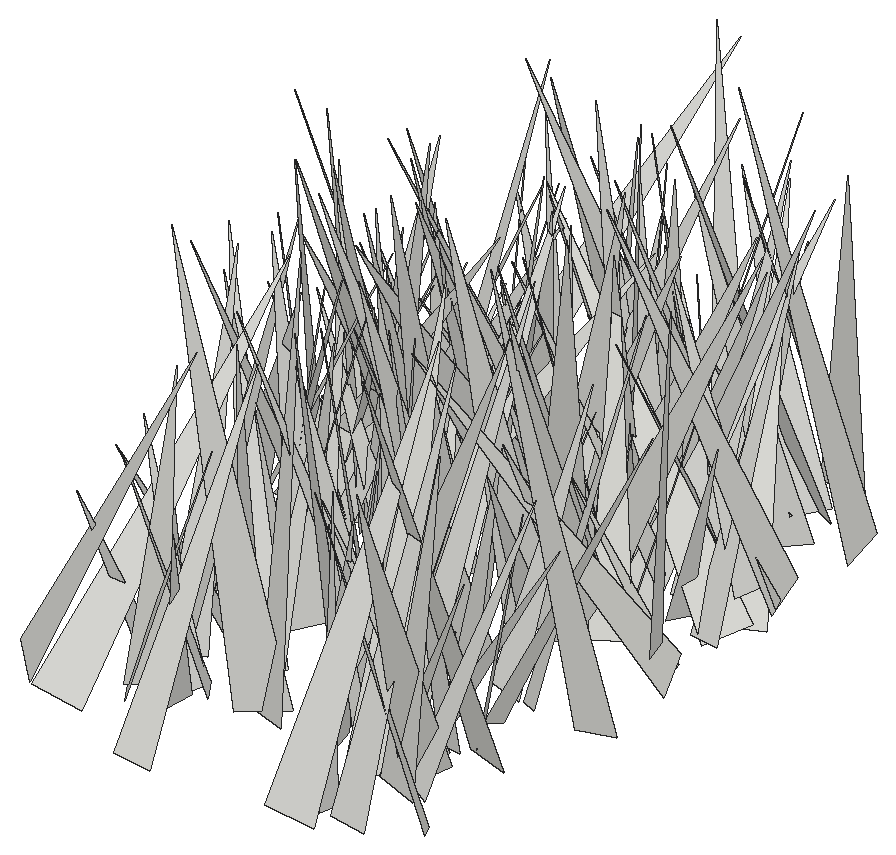
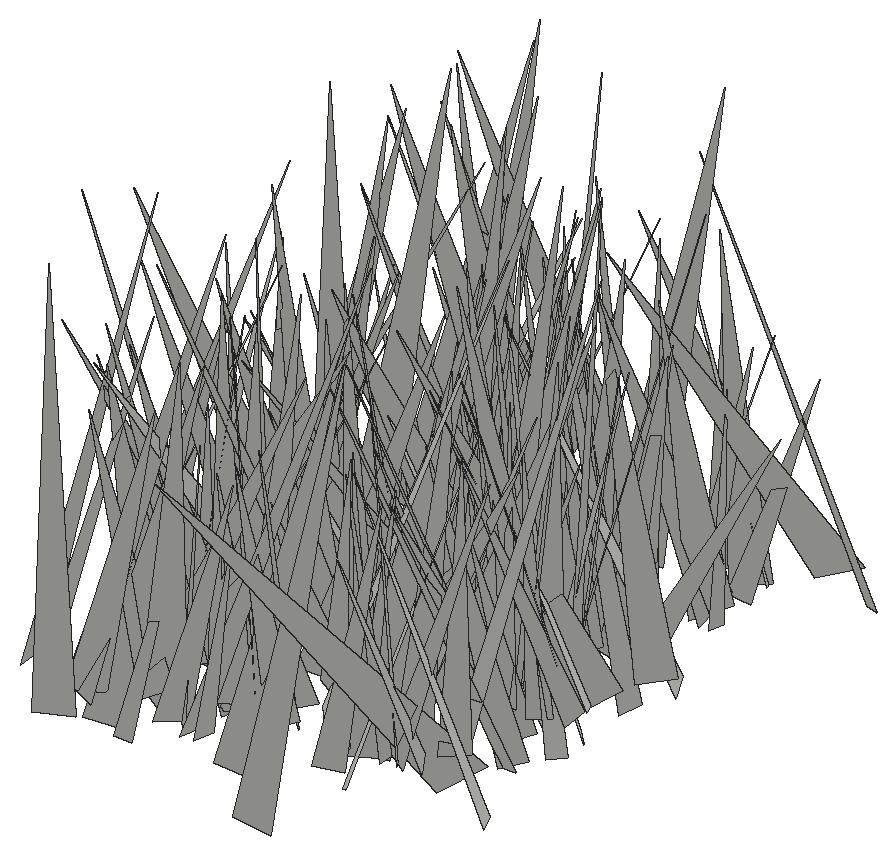
# SketchUp Ruby script. Lengths in inches.
U = 1.inch
M = Sketchup.active_model
def pt(a) = Geom::Point3d.new(a.map { |v| v * U })
def face(e, loops, mat)
  f = e.add_face(loops[0].map { |a| pt(a) })
  loops[1..].each { |l| e.add_face(l.map { |a| pt(a) }).erase! }
  f.material = f.back_material = mat if mat
  f
end
# faces: each face lists its corners as indices into pts; further lists are holes
def faces(e, pts, list, mat = nil) = list.each { |f| face(e, (f[0].is_a?(Array) ? f : [f]).map { |l| l.map { |i| pts[i] } }, mat) }
# xy, xz, yz: faces in a plane at the given z, y or x. An outline is a flat list of corners, or four numbers for a rectangle; further outlines are holes
def ring(l) = l.size == 4 ? [[l[0], l[1]], [l[2], l[1]], [l[2], l[3]], [l[0], l[3]]] : l.each_slice(2).to_a
def flat(e, list, mat, &to3) = list.each { |f| face(e, (f[0].is_a?(Array) ? f : [f]).map { |l| ring(l).map { |u, v| to3.(u, v) } }, mat) }
def xy(e, z, list, mat = nil) = flat(e, list, mat) { |x, y| [x, y, z] }
def xz(e, y, list, mat = nil) = flat(e, list, mat) { |x, z| [x, y, z] }
def yz(e, x, list, mat = nil) = flat(e, list, mat) { |y, z| [x, y, z] }
def lines(e, pts, list) = list.each { |a, b| e.add_line(pt(pts[a]), pt(pts[b])) }
# prism: a flat outline (further loops are holes) pulled along v
def prism(e, loops, v, mat = nil)
  f = face(e, loops, mat); d = Geom::Vector3d.new(v.map { |x| x * U })
  f.pushpull(f.normal.samedirection?(d) ? d.length : -d.length)
end
def box(e, o, s, mat = nil) = prism(e, [[o, [o[0] + s[0], o[1], o[2]], [o[0] + s[0], o[1] + s[1], o[2]], [o[0], o[1] + s[1], o[2]]]], [0, 0, s[2]], mat)
def at(x, y, z, deg = 0) = Geom::Transformation.translation(pt([x, y, z])) * Geom::Transformation.rotation(ORIGIN, Z_AXIS, deg.degrees)
def axes(o, x, y, z) = Geom::Transformation.new([*x, 0, *y, 0, *z, 0, *pt(o).to_a, 1])
def part(name) = M.definitions.add(name)
# library, detail: a bought-in or finely detailed component or shape, given as its bounding box
def library(name, o, s) = part(name).tap { |d| box(d.entities, o, s) }
def detail(e, o, s) = box(e.add_group.entities, o, s)
def put(e, d, t, mat = nil) = e.add_instance(d, t).tap { |i| i.material = mat if mat }
def group(e, t, mat = nil) = e.add_group.tap { |g| g.transformation = t; g.material = mat if mat }.entities
root = M.entities
c1 = part("fur_instance\#9")
p = [[0.8125,0,1.79],[0.67,-0.02,1.48],[0,-0.11,0],[0,0.11,0]]
faces(c1.entities,p,[[0,1,2,3]])
put(root,c1,axes([100.98,190.09,-27.1],[-2.4507,-4.58404,1.24543],[-4.71435,2.17524,-1.27033],[-0.58261,1.68089,5.0404]))
put(root,c1,axes([100.875,177.61,-28.22],[-0.33006,-3.76044,0.39687],[-3.50265,0.15395,-1.45434],[-1.42474,0.49269,3.4835]))
put(root,c1,axes([100.43,182.3,-28.22],[3.89411,3.28531,3.07479],[3.51498,-4.75969,0.63397],[-2.80935,-1.40135,5.05524]))
put(root,c1,axes([100.59,187.69,-28.22],[-4.98525,-6.36904,1.05647],[-6.36247,5.07321,0.56124],[1.09531,0.48105,8.06861]))
put(root,c1,axes([100.27,174.66,-28.22],[0.67909,-3.62862,0.46379],[-3.53581,-0.77205,-0.86319],[-0.93808,0.2832,3.58928]))
put(root,c1,axes([100.42,183.74,-27.1],[-4.38445,3.57185,1.79964],[3.76738,4.58485,0.07863],[1.34299,-1.20052,5.65467]))
put(root,c1,axes([100.8125,183.89,-27.1],[-6.07164,-2.28107,2.04855],[-2.55827,6.27412,-0.5961],[1.68971,1.3026,6.45854]))
put(root,c1,axes([100.88,179.83,-28.22],[-0.52973,-5.32119,2.08202],[-5.65742,0.19488,-0.94137],[-0.8022,2.1395,5.26399]))
put(root,c1,axes([100.17,184.2,-28.22],[-3.60567,-4.25836,0.82426],[-4.10665,3.69659,1.13335],[1.39586,-0.12438,5.46351]))
put(root,c1,axes([97.62,189.9,-28.22],[5.05169,2.87341,0.23488],[2.86098,-4.93803,-1.1233],[0.35552,-1.09113,5.70213]))
put(root,c1,axes([100.38,175.82,-28.22],[-5.11212,3.73872,1.49873],[3.53116,5.32488,-1.23875],[1.93782,0.15985,6.21106]))
put(root,c1,axes([98.25,184.95,-27.1],[4.49912,0.07902,0.02983],[0.07502,-4.46879,0.52292],[-0.03881,0.52233,4.46932]))
put(root,c1,axes([99.66,188.87,-27.1],[-3.20699,2.34244,2.63387],[2.95903,3.72406,0.29089],[1.91533,-1.83124,3.96071]))
put(root,c1,axes([99.71,176.41,-28.22],[3.54062,0.10617,1.20258],[0.38468,-3.63127,-0.812],[-1.14433,-0.89222,3.44788]))
put(root,c1,axes([97.8,181.64,-27.1],[2.89446,-5.47209,0.08006],[-5.31049,-2.7865,1.53693],[1.32243,0.78724,5.99662]))
put(root,c1,axes([99.11,185.56,-27.1],[1.24719,-3.91493,0.4967],[-3.8954,-1.13791,0.81231],[0.63182,0.71228,4.02769]))
put(root,c1,axes([96.81,172.67,-28.22],[5.1253,5.35023,0.94765],[5.22805,-4.50107,-2.86349],[1.48003,-2.62814,6.83331]))
put(root,c1,axes([102.79,176.58,-28.22],[-1.83761,6.5724,0.07775],[6.30696,1.74042,1.94227],[-1.85059,-0.59481,6.54223]))
put(root,c1,axes([100.66,182.59,-28.22],[-6.12859,-4.53414,1.24355],[-3.97845,6.08997,2.59781],[2.50535,-1.42065,7.16724]))
put(root,c1,axes([98.93,171.52,-28.22],[-2.37553,7.32496,0.20013],[6.77476,2.27563,-2.87444],[2.79244,0.71043,7.14393]))
put(root,c1,axes([99.67,183.23,-27.1],[6.5233,2.37968,3.04495],[3.30026,-6.53866,-1.96019],[-2.01069,-3.01183,6.66138]))
put(root,c1,axes([100.63,181.82,-27.1],[-2.63101,2.88231,1.12737],[2.88894,2.81797,-0.46255],[1.11028,-0.50218,3.87505]))
put(root,c1,axes([100.39,175.6,-28.22],[6.48387,0.57283,2.72889],[-0.5216,-6.53637,2.61139],[-2.73914,2.60063,5.96233]))
put(root,c1,axes([100.08,189.85,-27.1],[3.50829,2.33455,0.59392],[2.17247,-3.51961,1.00185],[-1.04078,0.52272,4.09323]))
put(root,c1,axes([100.02,185.17,-28.22],[-2.24113,2.46388,1.48853],[2.36542,2.65133,-0.82724],[1.6405,-0.45695,3.22631]))
put(root,c1,axes([98.65,184.1,-28.22],[4.58071,3.98416,0.78034],[4.05613,-4.44078,-1.1369],[0.17387,-1.36793,5.96354]))
put(root,c1,axes([98.3,179.92,-28.22],[5.74165,3.30721,0.02247],[3.30582,-5.73764,-0.2359],[0.09829,-0.21562,6.62182]))
put(root,c1,axes([98.36,184.14,-27.1],[4.34126,2.62004,0.01209],[2.52851,-4.18338,-1.34808],[0.68659,-1.1602,4.88813]))
put(root,c1,axes([102.34,183.51,-28.22],[-4.67838,0.58429,0.4377],[0.60816,4.68963,0.24018],[0.40387,-0.29353,4.7086]))
put(root,c1,axes([98.58,181.91,-28.22],[6.48852,0.93317,0.66882],[1.0636,-6.33108,-1.48501],[-0.43231,-1.57025,6.38486]))
put(root,c1,axes([101.82,174.375,-28.22],[-4.10178,1.61092,0.95507],[1.70987,4.15942,0.32775],[0.76391,-0.66031,4.39457]))
put(root,c1,axes([100.35,185.52,-27.1],[-1.33091,-4.34516,1.37723],[-4.35803,1.6335,0.94222],[1.33595,0.99989,4.44566]))
put(root,c1,axes([98.46,185.55,-28.22],[6.70588,0.95076,0.50826],[1.07552,-6.12086,-2.74035],[-0.07444,-2.78609,6.19381]))
put(root,c1,axes([101.58,183.73,-28.22],[-4.04138,0.55951,1.25439],[0.25517,4.13619,-1.02282],[1.34961,0.89343,3.94964]))
put(root,c1,axes([101.98,186.08,-27.1],[0.91658,-6.09487,0.23316],[-5.96683,-0.94489,-1.24341],[-1.26442,0.04079,6.03668]))
put(root,c1,axes([100.53,173.76,-28.22],[3.55242,-4.27149,1.91187],[-4.60398,-3.6203,0.46613],[-0.83917,1.77997,5.53606]))
put(root,c1,axes([100.52,181.37,-27.1],[3.76138,-1.24538,0.93866],[-1.27843,-3.86595,-0.00634],[-0.89313,0.28885,3.96218]))
put(root,c1,axes([102.1875,174.68,-28.22],[-3.61255,-2.36918,0.54232],[-2.35627,3.65218,0.25916],[0.59592,0.07847,4.31235]))
put(root,c1,axes([99.2,186.66,-28.22],[1.64693,-4.65446,0.85777],[-4.4282,-1.19483,2.01879],[1.67056,1.42146,4.50564]))
put(root,c1,axes([100.32,183.96,-27.1],[-1.02594,6.32348,2.52203],[6.58274,1.57191,-1.26344],[1.73626,-2.22313,6.28034]))
put(root,c1,axes([101.61,185.42,-27.1],[-1.56855,-7.63886,0.47282],[-7.63369,1.59619,0.46371],[0.55001,0.36889,7.78444]))
put(root,c1,axes([102.1,191.83,-27.1],[1.8151,-3.86013,1.55176],[-3.9232,-2.15155,-0.76319],[-1.38458,1.03602,4.19675]))
put(root,c1,axes([102.1875,179.7,-28.22],[-5.43342,3.18473,2.47254],[3.60205,5.6984,0.57576],[1.81141,-1.77869,6.27161]))
put(root,c1,axes([98.34,183.59,-27.1],[4.70359,-4.43483,0.77561],[-4.1988,-3.91632,3.07011],[1.62462,2.71804,5.6891]))
put(root,c1,axes([103.16,185.85,-27.1],[-3.34237,-3.67886,0.49489],[-3.71061,3.29315,-0.58039],[-0.10119,0.75599,4.93646]))
put(root,c1,axes([100.68,184.72,-28.22],[-0.26739,4.57604,0.32256],[4.40279,0.34673,-1.26925],[1.2883,-0.2352,4.40462]))
put(root,c1,axes([100.87,190.08,-27.1],[4.61711,2.95667,1.94744],[3.35791,-4.67134,-0.86895],[-1.12198,-1.8135,5.41336]))
put(root,c1,axes([103.87,185.64,-27.1],[-0.77186,4.35622,1.72795],[4.2436,-0.09339,2.13104],[-1.98854,-1.8902,3.87699]))
put(root,c1,axes([100.25,180.17,-28.22],[5.36268,3.16176,1.79895],[3.56295,-5.21159,-1.4615],[-0.73371,-2.1986,6.05138]))
put(root,c1,axes([101.04,185.3,-27.1],[-1.24529,-7.71146,0.7872],[-7.61167,1.36728,1.35282],[1.46589,0.54863,7.69333]))
put(root,c1,axes([100.09,182.55,-28.22],[2.55836,5.15566,0.46861],[5.11042,-2.43162,-1.14739],[0.82709,-0.92305,5.63999]))
put(root,c1,axes([99.83,188.29,-28.22],[-4.06981,7.2471,0.38585],[5.9474,3.58401,-4.58433],[4.15906,1.9665,6.9331]))
put(root,c1,axes([100.18,173.33,-28.22],[4.57096,2.53062,0.74602],[2.63797,-4.36083,-1.37058],[0.04077,-1.55993,5.04174]))
put(root,c1,axes([99.12,186.99,-28.22],[3.70489,5.29932,0.63458],[5.07029,-3.25343,-2.43293],[1.66665,-1.88258,5.99082]))
put(root,c1,axes([101.12,183.57,-27.1],[-2.2184,-4.85625,2.50772],[-5.03427,2.86928,1.10295],[2.1279,1.72546,5.22379]))
put(root,c1,axes([101.44,183.625,-28.22],[6.98669,-0.82296,2.45735],[-1.02769,-7.36659,0.45485],[-2.37901,0.76535,7.02027]))
put(root,c1,axes([101.55,177.47,-28.22],[-1.49561,-5.63035,1.67127],[-5.71638,1.79132,0.91926],[1.34798,1.34949,5.75262]))
put(root,c1,axes([102.22,190.92,-28.22],[-3.99829,-3.957,0.07334],[-3.50173,3.58563,2.55553],[1.84422,-1.77059,5.01133]))
put(root,c1,axes([101.11,190.28,-27.1],[4.30698,0.82715,0.77594],[0.97071,-4.26434,-0.84231],[-0.5865,-0.98365,4.30404]))
put(root,c1,axes([101.54,178.26,-28.22],[4.69636,2.95892,0.9191],[2.85112,-4.78039,0.82137],[-1.21287,0.21986,5.48965]))
put(root,c1,axes([102.53,184.15,-27.1],[3.62911,6.60842,0.2466],[6.35712,-3.56375,1.94657],[-1.82181,0.72867,7.28371]))
put(root,c1,axes([101.15,189.01,-27.1],[5.45875,-2.61976,0.1584],[-2.41646,-5.15945,-2.05595],[-1.02417,-1.78972,5.6951]))
put(root,c1,axes([101.06,185.93,-27.1],[1.63148,3.88333,0.8996],[3.80186,-1.22375,-1.61232],[1.19808,-1.40479,3.89132]))
put(root,c1,axes([102.97,194.36,-28.22],[-1.0754,-7.3325,1.08617],[-7.40599,1.10888,0.15329],[0.31086,1.05196,7.40935]))
put(root,c1,axes([101.9375,173.57,-28.22],[3.94789,-1.4658,0.35037],[-1.34081,-3.86465,-1.06014],[-0.68816,-0.87925,4.0756]))
put(root,c1,axes([104.23,174.6875,-28.22],[2.49125,-7.31611,3.2771],[-7.62751,-3.2193,-1.38865],[-2.46697,2.5655,7.60286]))
put(root,c1,axes([103.25,188.63,-27.1],[-1.22069,-3.41408,1.05948],[-3.55821,1.26785,-0.01408],[0.34288,1.00256,3.62571]))
put(root,c1,axes([103.94,184.47,-28.22],[-7.41474,-1.37074,2.09218],[-0.74138,7.45582,2.25736],[2.38883,-1.94072,7.19456]))
put(root,c1,axes([104.77,188.24,-27.1],[1.00631,5.78428,1.17144],[5.41169,-1.37849,2.15781],[-2.35451,-0.6962,5.46025]))
put(root,c1,axes([104.25,189.35,-27.1],[-5.79035,-4.99721,0.36352],[-4.82955,5.71454,1.62848],[1.33407,-1.00217,7.47317]))
put(root,c1,axes([103.11,188.89,-28.22],[2.31085,-7.14722,0.11909],[-7.10013,-2.30949,-0.83147],[-0.82765,-0.14321,7.46535]))
put(root,c1,axes([103.4,184.15,-27.1],[-5.97447,-2.65496,2.2585],[-2.10106,6.3191,1.8704],[2.78122,-0.92951,6.26456]))
put(root,c1,axes([104.46,185.94,-27.1],[-2.38494,-6.16406,1.52656],[-6.35023,2.30898,-0.59758],[-0.0234,1.63919,6.58229]))
put(root,c1,axes([103.66,184.99,-28.22],[1.41164,-4.04262,0.99191],[-4.10193,-1.52908,-0.39425],[-0.70768,0.79907,4.26381]))
put(root,c1,axes([103.11,169.86,-28.22],[0.40052,6.46259,0.29319],[6.45769,-0.38185,-0.40475],[0.38629,-0.31712,6.46233]))
put(root,c1,axes([104.18,181.32,-28.22],[-6.58404,0.20466,2.39247],[0.20033,7.00521,-0.04793],[2.39284,-0.02336,6.58705]))
put(root,c1,axes([103.93,182.38,-27.1],[-0.42673,3.51272,1.26133],[3.73148,0.37463,0.21911],[-0.0791,-1.27778,3.53176]))
put(root,c1,axes([104.52,182.29,-28.22],[-3.06168,2.49465,0.02952],[2.42804,2.99025,-0.87237],[0.57338,0.65813,3.85176]))
put(root,c1,axes([103.3125,188.57,-27.1],[-0.92871,-3.83483,1.6083],[-4.04735,1.2119,0.55253],[0.95473,1.40727,3.90681]))
put(root,c1,axes([103.21,181.43,-27.1],[-0.85161,3.55792,0.87868],[3.50079,1.05663,-0.88551],[1.08413,-0.61714,3.54963]))
put(root,c1,axes([103.71,175.39,-28.22],[-0.34341,4.80516,0.97397],[4.88667,0.41477,-0.32328],[0.39826,-0.94579,4.80656]))
put(root,c1,axes([104.87,182.89,-27.1],[-1.89303,-4.40404,0.51291],[-4.43222,1.86471,-0.34716],[-0.11875,0.60786,4.78107]))
put(root,c1,axes([103.73,182.01,-27.1],[3.9323,-0.29865,1.47953],[-0.48436,-4.16008,0.44758],[-1.42954,0.58799,3.91814]))
put(root,c1,axes([104.73,174.36,-28.22],[2.9733,6.47594,2.08154],[6.51847,-3.36189,1.14821],[-1.94427,-1.36785,7.03277]))
put(root,c1,axes([105.08,185.48,-27.1],[-3.3946,-3.12525,1.18102],[-3.29173,3.41661,-0.4203],[0.5714,1.11577,4.59499]))
put(root,c1,axes([104.89,191.37,-28.22],[-1.62958,-3.15436,1.09529],[-3.33909,1.53504,-0.54711],[-0.01197,1.22427,3.50802]))
put(root,c1,axes([103.59,187.29,-28.22],[3.65469,-1.69105,0.3912],[-1.57801,-3.61693,-0.89287],[-0.72291,-0.65395,3.92673]))
put(root,c1,axes([104.39,187.56,-27.1],[6.48177,-5.01878,0.45242],[-4.24735,-5.8379,-3.90962],[-2.71162,-2.85253,7.2053]))
put(root,c1,axes([103.65,183.98,-27.1],[7.48346,-2.4752,1.75576],[-1.96533,-7.51292,-2.21472],[-2.31232,-1.62508,7.56464]))
put(root,c1,axes([102.9375,189.04,-28.22],[0.69431,-7.1025,1.01226],[-6.95299,-0.41552,1.85354],[1.7681,1.15502,6.89145]))
put(root,c1,axes([107.34,177.13,-28.22],[-6.50715,-2.26194,0.29712],[-2.26712,6.51165,-0.07913],[0.25462,0.17236,6.88863]))
put(root,c1,axes([106.64,192.5,-27.1],[-7.7703,-1.5883,1.42664],[-1.2052,7.70803,2.01725],[1.76224,-1.7318,7.67014]))
put(root,c1,axes([106.3,188.24,-28.22],[3.23969,5.31398,1.47982],[4.81259,-3.56155,2.25346],[-2.69577,0.02794,5.80137]))
put(root,c1,axes([104.8125,190.59,-27.1],[3.28542,-2.52777,1.83261],[-2.97263,-3.34603,0.71392],[-0.95477,1.71946,4.08337]))
put(root,c1,axes([105.97,187.58,-27.1],[2.24091,-5.47361,0.67385],[-5.23088,-2.33999,-1.61199],[-1.7471,-0.01469,5.69066]))
put(root,c1,axes([102.41,183.83,-27.1],[0.90469,6.24799,0.05202],[5.52251,-0.775,-2.9597],[2.92267,-0.46962,5.57638]))
put(root,c1,axes([105.51,192.12,-28.22],[-0.44109,-6.89492,0.21564],[-6.89758,0.44393,0.08524],[0.09888,0.20974,6.90849]))
put(root,c1,axes([103.32,182.65,-27.1],[4.26257,2.91433,0.00484],[2.86478,-4.18851,-0.95515],[0.53516,-0.79116,5.0745]))
put(root,c1,axes([105.51,183.45,-28.22],[4.42049,5.15695,1.86392],[5.12768,-4.73588,0.94203],[-1.94301,-0.76574,6.72662]))
put(root,c1,axes([106.2,192.6,-27.1],[-3.46887,0.5768,0.94943],[0.60796,3.5911,0.03958],[0.92978,-0.19616,3.51628]))
put(root,c1,axes([105.18,179.75,-28.22],[-3.24328,-4.06122,2.56752],[-4.33534,3.80899,0.54855],[2.07134,1.61325,5.16831]))
put(root,c1,axes([106.83,177.11,-28.22],[-5.04486,-3.51647,1.75014],[-3.733,5.17856,-0.35556],[1.22196,1.30239,6.1392]))
put(root,c1,axes([106.33,186.18,-27.1],[-3.36385,-0.86607,1.07357],[-0.51946,3.41676,1.12873],[1.27781,-0.89095,3.28504]))
put(root,c1,axes([107.08,176.67,-28.22],[4.87258,-2.82126,2.84071],[-2.53321,-5.63755,-1.25383],[-3.10033,0.17232,5.48903]))
put(root,c1,axes([107.26,188.9,-28.22],[-7.11208,1.53537,2.26223],[1.65379,7.4363,0.15223],[2.17716,-0.6331,7.27433]))
put(root,c1,axes([106.5,179.08,-28.22],[-5.35866,5.61511,0.59327],[5.12673,5.1813,-2.73266],[2.36603,1.4904,7.2648]))
put(root,c1,axes([106.0625,176.23,-28.22],[-6.11732,-3.75265,2.76683],[-3.28898,6.70851,1.82699],[3.3046,-0.26993,6.94018]))
put(root,c1,axes([106.03,190.28,-27.1],[4.89735,3.35239,2.18214],[3.80193,-4.97328,-0.89225],[-1.24321,-2.00306,5.86741]))
put(root,c1,axes([104.39,187.86,-27.1],[3.12045,6.97557,0.92804],[6.87353,-2.80376,-2.03727],[1.5081,-1.6545,7.36514]))
put(root,c1,axes([107.09,180.84,-28.22],[3.52334,-7.25518,1.10129],[-7.15699,-3.66725,-1.26216],[-1.62106,0.42196,7.96608]))
put(root,c1,axes([108.79,190.91,-28.22],[-4.22119,3.06488,0.48562],[3.10212,4.18863,0.52921],[0.07866,-0.71394,5.1896]))
put(root,c1,axes([106.89,189.4,-28.22],[2.53545,-3.02814,1.98338],[-3.53036,-2.60371,0.53779],[-0.80002,1.89288,3.91266]))
put(root,c1,axes([108.73,173.99,-28.22],[0.33091,4.05955,1.18914],[3.81261,-0.80293,1.68011],[-1.83248,-0.93747,3.71034]))
put(root,c1,axes([109.18,190.84,-27.1],[-7.08431,2.74004,0.68893],[2.60293,7.0529,-1.28499],[1.09872,0.95845,7.48626]))
put(root,c1,axes([107.4,189.14,-28.22],[3.10657,-5.20372,2.6425],[-5.63717,-3.45056,-0.16782],[-1.51121,2.17421,6.05816]))
put(root,c1,axes([106.35,174.96,-28.22],[4.0424,-1.6774,0.68877],[-1.67315,-4.09915,-0.16314],[-0.69903,0.11126,4.37357]))
put(root,c1,axes([110.16,190.21,-28.22],[-2.5015,-6.23633,1.72664],[-6.18785,1.76379,-2.59425],[-1.89304,2.47545,6.19832]))
put(root,c1,axes([106.82,184.24,-28.22],[-1.9043,4.31856,1.08738],[4.14528,2.15112,-1.28374],[1.62757,-0.42591,4.54184]))
put(root,c1,axes([107.03,182.57,-28.22],[3.38702,2.66566,0.2184],[2.51461,-3.29384,1.20529],[-0.91115,0.81867,4.13823]))
put(root,c1,axes([109.69,186.85,-27.1],[-5.35424,-1.86738,0.02315],[-1.86377,5.3475,0.29345],[0.11847,-0.26947,5.66294]))
put(root,c1,axes([106.85,190.58,-27.1],[2.3512,-5.85332,1.44977],[-6.03015,-2.28819,0.5412],[-0.02311,1.54732,6.28463]))
put(root,c1,axes([107.2,174.72,-28.22],[4.4988,1.24272,1.44893],[1.33102,-4.70119,-0.10058],[-1.36826,-0.48722,4.6662]))
put(root,c1,axes([108.12,186.3,-27.1],[-3.94207,-4.94022,1.13908],[-4.81769,4.09962,1.10733],[1.57897,0.1748,6.2225]))
put(root,c1,axes([106.26,186.59,-27.1],[2.2039,-6.87435,1.74953],[-7.02125,-1.85328,1.56272],[1.00974,2.1174,7.04782]))
put(root,c1,axes([105.57,186.8,-27.1],[3.73995,-4.97965,1.07609],[-4.97131,-3.27521,2.12161],[1.114,2.10195,5.85517]))
put(root,c1,axes([108.37,186.8125,-28.22],[6.19858,3.66698,3.16063],[3.75526,-6.8827,0.6206],[-3.05522,-1.01998,7.17523]))
put(root,c1,axes([110.29,188.8,-28.22],[-4.58076,1.47717,0.18742],[1.47131,4.39705,1.30451],[-0.22897,-1.29786,4.63288]))
put(root,c1,axes([109.75,182.05,-27.1],[-6.16922,0.32467,1.04524],[-0.06119,5.87189,-2.18505],[1.09279,2.16166,5.77844]))
put(root,c1,axes([108.41,190.86,-28.22],[-3.07228,-3.20464,1.70758],[-3.41257,3.31254,0.07678],[1.24093,1.17551,4.43878]))
put(root,c1,axes([109.81,189.1,-28.22],[-5.99226,-3.56649,1.99916],[-3.93709,5.99,-1.11487],[1.10264,2.00593,6.88361]))
put(root,c1,axes([109.97,176.35,-28.22],[1.91991,5.69676,2.84026],[5.7974,-2.78995,1.67703],[-2.62873,-1.9923,5.77292]))
put(root,c1,axes([112.11,186.86,-28.22],[-5.51381,4.9525,0.02994],[4.6746,5.18943,2.47955],[-1.63592,-1.86355,6.98435]))
put(root,c1,axes([107.17,188.2,-27.1],[1.92624,-6.27783,0.49509],[-6.26935,-1.863,0.76884],[0.59288,0.69623,6.52153]))
put(root,c1,axes([107.99,194.21,-27.1],[3.38324,-1.277,0.34003],[-0.90165,-2.91389,-1.97203],[-0.96612,-1.75247,3.03119]))
put(root,c1,axes([108.72,182.01,-27.1],[6.46231,-4.31648,2.52967],[-3.92803,-6.93665,-1.8017],[-3.09867,-0.20881,7.55958]))
put(root,c1,axes([110.46,183.51,-27.1],[-2.82559,-5.19892,1.36333],[-5.31081,2.46391,-1.61114],[-0.82624,1.9421,5.69358]))
put(root,c1,axes([107.96,179.41,-28.22],[4.13039,-0.87619,1.21239],[-0.99071,-4.26996,0.28929],[-1.12075,0.54542,4.21238]))
put(root,c1,axes([107.96,176.8,-28.22],[1.83288,7.01444,0.75411],[7.05484,-1.82448,-0.17632],[-0.01908,-0.77421,7.24781]))
put(root,c1,axes([109.45,171.26,-28.22],[-4.70779,-0.34884,1.44292],[-0.70643,4.74641,-1.15738],[1.30563,1.3103,4.57662]))
put(root,c1,axes([110.33,175.54,-28.22],[-4.68733,-0.90911,0.30449],[-0.85582,4.65242,0.7161],[0.43216,-0.64711,4.72067]))
put(root,c1,axes([109.15,173.73,-28.22],[-5.06165,5.7028,1.49455],[5.55918,5.27278,-1.292],[1.96243,-0.22764,7.51486]))
put(root,c1,axes([110.2,192.26,-28.22],[-3.08305,4.83073,2.80211],[5.58378,2.72141,1.452],[0.09585,-3.15451,5.54372]))
put(root,c1,axes([108.44,182.3125,-27.1],[4.1039,-1.37964,0.4984],[-1.03776,-3.77714,-1.91052],[-1.03675,-1.68037,3.88527]))
put(root,c1,axes([110.67,192.62,-27.1],[-3.89894,3.87426,1.21258],[4.05705,3.77806,0.97396],[0.14352,-1.54866,5.40953]))
put(root,c1,axes([108.96,189.11,-27.1],[3.6892,-1.49713,1.29137],[-1.47127,-3.90506,-0.32413],[-1.32076,0.16824,3.96818]))
put(root,c1,axes([106.39,187.95,-28.22],[2.05152,-6.6713,2.37008],[-6.64568,-0.96384,3.03943],[2.44098,2.98279,6.28306]))
put(root,c1,axes([106.97,175.6875,-28.22],[6.69732,-3.52244,1.21858],[-3.71872,-6.48437,1.69431],[-0.25228,2.07171,7.37503]))
put(root,c1,axes([107.73,184.48,-27.1],[5.80631,-5.6916,0.53269],[-5.68589,-5.82856,-0.29992],[-0.59055,0.15799,8.12513]))
put(root,c1,axes([107.61,189.03,-28.22],[5.04993,-3.13211,0.88061],[-3.25342,-4.87587,1.31476],[-0.02926,1.58216,5.79512]))
put(root,c1,axes([110.32,184.45,-27.1],[5.94606,5.36025,0.59468],[4.2161,-5.17199,4.4628],[-3.36309,2.9933,6.64615]))
put(root,c1,axes([110.77,192.84,-27.1],[-3.23676,-6.95107,0.75182],[-6.9834,3.25434,0.02332],[0.33861,0.67166,7.66769]))
put(root,c1,axes([109.88,182.07,-28.22],[2.52886,2.74781,0.4271],[2.47453,-2.48701,1.34889],[-1.2687,0.62635,3.48225]))
put(root,c1,axes([108.9,191.46,-27.1],[4.04203,-2.33275,1.48439],[-2.65208,-4.01454,0.91276],[-0.78205,1.55722,4.57675]))
put(root,c1,axes([108.84,184.39,-28.22],[6.98894,-3.62557,1.01436],[-3.15649,-6.80873,-2.58782],[-2.05189,-1.87497,7.43594]))
put(root,c1,axes([108.83,170.2,-28.22],[-0.59068,7.87895,1.19707],[7.83923,0.79048,-1.33468],[1.43434,-1.07565,7.78752]))
put(root,c1,axes([110.84,182.89,-27.1],[-3.10471,5.12305,0.88051],[5.18598,3.12286,0.11631],[0.35573,-0.81381,5.98927]))
put(root,c1,axes([109.1,180.06,-28.22],[0.7475,5.23214,1.319],[5.34274,-0.53135,-0.92008],[0.75507,-1.41992,5.20456]))
put(root,c1,axes([108.9375,173.82,-28.22],[6.03648,4.13261,1.07509],[4.02235,-6.12795,0.97074],[-1.43354,0.20766,7.25088]))
put(root,c1,axes([112.58,172.02,-28.22],[-4.67684,-2.75,0.36196],[-2.71074,4.38122,-1.73872],[-0.58771,1.67594,5.13928]))
put(root,c1,axes([110.18,183.02,-27.1],[4.14247,-2.36814,0.94959],[-1.79033,-3.98803,-2.13546],[-1.81783,-1.46881,4.26707]))
put(root,c1,axes([110,187.65,-28.22],[1.00933,7.00307,0.82634],[7.04916,-1.02422,0.06983],[-0.18746,-0.80782,7.07509]))
put(root,c1,axes([110.19,179.84,-28.22],[3.77258,4.9169,0.38845],[4.64704,-3.70729,1.79444],[-1.65279,0.7995,5.93196]))
put(root,c1,axes([112.36,183.93,-28.22],[-7.29463,-2.71144,0.02018],[-2.47986,6.69465,3.09773],[1.09665,-2.89718,7.13916]))
put(root,c1,axes([108.79,186.55,-28.22],[1.06363,7.1406,0.14161],[6.98782,-1.01087,-1.51263],[1.47601,-0.35985,7.05914]))
put(root,c1,axes([113.24,187.98,-27.1],[-6.30191,-3.29477,0.26908],[-3.30318,6.25333,-0.79169],[-0.13009,0.82599,7.06702]))
put(root,c1,axes([108.9,177.35,-28.22],[3.6219,-1.04912,0.12415],[-1.02885,-3.40219,1.26523],[0.23987,1.24847,3.55218]))
put(root,c1,axes([110.48,170.86,-28.22],[1.7832,7.11152,0.69499],[7.11724,-1.83129,0.47737],[-0.63379,-0.55606,7.31612]))
put(root,c1,axes([111.29,176.49,-28.22],[-2.16653,-7.31637,0.90738],[-7.36569,2.18851,0.05952],[0.3151,0.85299,7.63018]))
put(root,c1,axes([109.5,174.13,-28.22],[3.74369,-0.67268,0.40161],[-0.71907,-3.7286,0.45768],[-0.31101,0.52348,3.776]))
put(root,c1,axes([110.15,189.18,-27.1],[-3.50557,-5.51536,0.11612],[-4.95597,3.20905,2.80393],[2.42302,-1.41579,5.90306]))
put(root,c1,axes([112.25,184.09,-28.22],[-3.53813,-0.73541,0.01575],[-0.72603,3.50386,0.50526],[0.11809,-0.49152,3.57826]))
put(root,c1,axes([112.125,192.93,-27.1],[-3.86878,-4.9807,0.99535],[-5.05831,3.89149,-0.18804],[0.45997,0.9025,6.30392]))
put(root,c1,axes([112.28,187.84,-27.1],[-4.9541,1.83691,1.27432],[2.05779,4.95762,0.85363],[0.87385,-1.26054,5.21428]))
put(root,c1,axes([112.1875,187.43,-28.22],[-3.69849,5.78351,0.10997],[5.76561,3.69627,-0.48502],[0.46777,0.16892,6.84781]))
put(root,c1,axes([110.43,177.23,-28.22],[3.70099,1.78589,1.07617],[1.91017,-3.78303,-0.29128],[-0.83593,-0.7377,4.09901]))
put(root,c1,axes([112.79,179.78,-28.22],[-1.04276,-7.37455,2.60053],[-7.71345,0.53914,-1.56404],[-1.28435,2.74945,7.28184]))
put(root,c1,axes([110.01,178.41,-28.22],[5.03908,0.51167,0.65236],[0.18588,-4.61324,2.18248],[-0.80798,2.12978,4.57066]))
put(root,c1,axes([110.32,186.77,-28.22],[3.31097,-1.72543,0.32906],[-1.73993,-3.31791,0.10944],[-0.24091,0.24944,3.73197]))
put(root,c1,axes([110.55,174.59,-28.22],[5.9537,-4.05045,0.58701],[-3.75603,-5.81897,-2.05648],[-1.62572,-1.38951,6.90098]))
put(root,c1,axes([108.55,188.55,-27.1],[4.54413,5.8348,1.67226],[5.93472,-3.83302,-2.75273],[1.27295,-2.95864,6.86415]))
put(root,c1,axes([108.95,183.99,-27.1],[5.79439,-3.93356,1.43708],[-4.17619,-5.2444,2.48372],[0.31237,2.85246,6.54821]))
put(root,c1,axes([110.3,173.4375,-28.22],[1.5633,5.69815,3.01797],[6.40687,-1.02237,-1.38843],[0.72737,-3.24142,5.74326]))
put(root,c1,axes([113.22,188.19,-27.1],[-7.42684,-1.75978,1.28146],[-1.36577,7.3143,2.12899],[1.69519,-1.81689,7.32954]))
put(root,c1,axes([111.79,186.15,-28.22],[1.80185,5.93958,0.37976],[5.89361,-1.83593,0.75111],[-0.82954,-0.14229,6.16126]))
put(root,c1,axes([113.23,191.85,-27.1],[-7.82049,-1.65264,1.82204],[-1.48703,8.01344,0.88582],[1.95953,-0.51451,7.94397]))
put(root,c1,axes([110.52,194.31,-27.1],[1.17808,-6.7396,1.1437],[-6.76699,-0.98532,1.16408],[0.96855,1.31342,6.74203]))
put(root,c1,axes([112.29,183.24,-27.1],[-4.83531,-1.63891,2.39644],[-2.01972,5.24312,-0.48946],[2.08559,1.27782,5.08199]))
put(root,c1,axes([110.77,173.78,-28.22],[2.45412,4.72767,0.6627],[4.74881,-2.3413,-0.8831],[0.48874,-0.99004,5.25297]))
